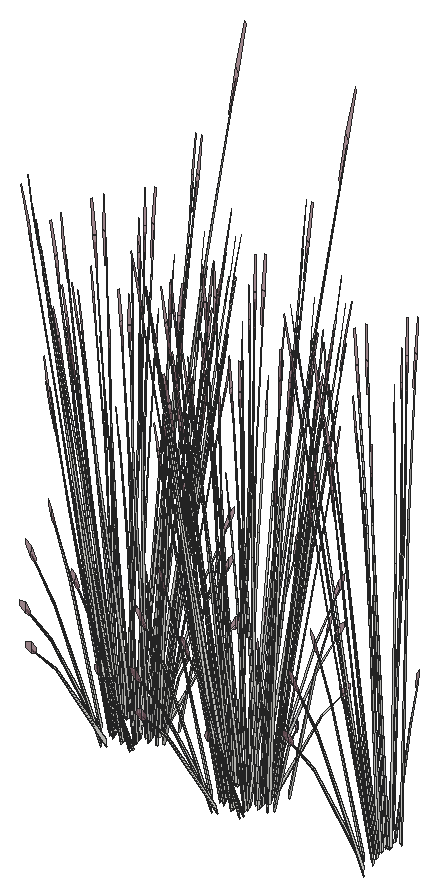
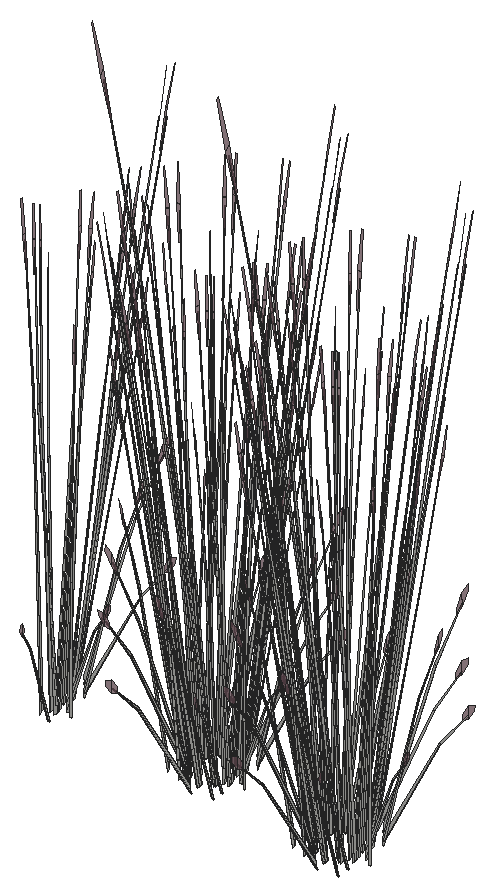
# SketchUp Ruby script. Lengths in inches.
U = 1.inch
M = Sketchup.active_model
def pt(a) = Geom::Point3d.new(a.map { |v| v * U })
def face(e, loops, mat)
  f = e.add_face(loops[0].map { |a| pt(a) })
  loops[1..].each { |l| e.add_face(l.map { |a| pt(a) }).erase! }
  f.material = f.back_material = mat if mat
  f
end
# faces: each face lists its corners as indices into pts; further lists are holes
def faces(e, pts, list, mat = nil) = list.each { |f| face(e, (f[0].is_a?(Array) ? f : [f]).map { |l| l.map { |i| pts[i] } }, mat) }
# xy, xz, yz: faces in a plane at the given z, y or x. An outline is a flat list of corners, or four numbers for a rectangle; further outlines are holes
def ring(l) = l.size == 4 ? [[l[0], l[1]], [l[2], l[1]], [l[2], l[3]], [l[0], l[3]]] : l.each_slice(2).to_a
def flat(e, list, mat, &to3) = list.each { |f| face(e, (f[0].is_a?(Array) ? f : [f]).map { |l| ring(l).map { |u, v| to3.(u, v) } }, mat) }
def xy(e, z, list, mat = nil) = flat(e, list, mat) { |x, y| [x, y, z] }
def xz(e, y, list, mat = nil) = flat(e, list, mat) { |x, z| [x, y, z] }
def yz(e, x, list, mat = nil) = flat(e, list, mat) { |y, z| [x, y, z] }
def lines(e, pts, list) = list.each { |a, b| e.add_line(pt(pts[a]), pt(pts[b])) }
# prism: a flat outline (further loops are holes) pulled along v
def prism(e, loops, v, mat = nil)
  f = face(e, loops, mat); d = Geom::Vector3d.new(v.map { |x| x * U })
  f.pushpull(f.normal.samedirection?(d) ? d.length : -d.length)
end
def box(e, o, s, mat = nil) = prism(e, [[o, [o[0] + s[0], o[1], o[2]], [o[0] + s[0], o[1] + s[1], o[2]], [o[0], o[1] + s[1], o[2]]]], [0, 0, s[2]], mat)
def at(x, y, z, deg = 0) = Geom::Transformation.translation(pt([x, y, z])) * Geom::Transformation.rotation(ORIGIN, Z_AXIS, deg.degrees)
def axes(o, x, y, z) = Geom::Transformation.new([*x, 0, *y, 0, *z, 0, *pt(o).to_a, 1])
def part(name) = M.definitions.add(name)
# library, detail: a bought-in or finely detailed component or shape, given as its bounding box
def library(name, o, s) = part(name).tap { |d| box(d.entities, o, s) }
def detail(e, o, s) = box(e.add_group.entities, o, s)
def put(e, d, t, mat = nil) = e.add_instance(d, t).tap { |i| i.material = mat if mat }
def group(e, t, mat = nil) = e.add_group.tap { |g| g.transformation = t; g.material = mat if mat }.entities
root = M.entities
M.materials.add("LightPink_Translucent").color = [144, 107, 117]
M.materials["LightPink_Translucent"].alpha = 0.75
c1 = part("blade")
p = [[2.15,0.21,22],[0,0.17,0],[0.09,0.45,0],[2.18,0.31,22],[2.29,0.31,22],[0.38,0.45,0],
  [2.48,0.24,33],[2.49,0.24,33],[2.48,0.22,33]]
faces(c1.entities,p,[[0,1,2,3],[4,5,2,3],[6,3,4,7],[8,0,3,6]])
c2 = part("seeds")
p = [[0.3,-0.1,1.38],[-0.01,-0.03,1.59],[-0.01,-0.03,0.03],[0.14,-0.07,-0.07],[0.29,-0.03,3],[0.15,0.01,3.11]]
faces(c2.entities,p,[[0,1,2,3],[1,0,4,5]],"LightPink_Translucent")
c3 = part("blade with seeds")
put(c3.entities,c1,at(0,0,0))
put(c3.entities,c2,axes([2.4,0.25,30.99],[1.5799,-0.05474,1.17369],[-0.12525,1.92788,0.29478],[-0.07173,-0.02425,1.56792]))
put(root,c3,axes([341.86,791.42,4.72],[-0.05763,0.06055,1.74944],[0.0049,0.44239,-0.27667],[-0.13211,0.05753,0.14031]))
put(root,c3,axes([341.22,791.87,4.71],[0.04504,0.01251,1.77383],[0.13934,0.41205,-0.16761],[-0.0922,0.10815,0.31391]))
put(root,c3,axes([342.13,789.58,4.71],[0.02617,0.04654,1.77383],[-0.12614,0.41836,-0.16761],[-0.12775,0.00303,0.31391]))
put(root,c3,axes([342.42,789.3,4.72],[-0.07594,-0.00329,1.74944],[-0.24177,0.32918,-0.27667],[-0.129,-0.06726,0.14031]))
put(root,c3,axes([342.11,791.12,4.73],[0.09971,-0.42522,0.48003],[0.32782,0.1454,0.3958],[-0.12892,0.02555,0.9933]))
put(root,c3,axes([342.23,791,5.03],[0.17758,0.42229,-0.1216],[-0.31518,0.20752,-0.67495],[-0.13282,0.05572,1.02557]))
put(root,c3,axes([342.63,790.12,5.03],[-0.0189,0.47427,-0.1216],[-0.35781,-0.01296,-0.67495],[-0.13781,-0.03295,1.02557]))
put(root,c3,axes([342.09,791.01,4.73],[-0.12963,-0.31798,0.0643],[0.23638,-0.15564,0.50621],[-0.1042,0.03071,0.77189]))
put(root,c3,axes([342.19,792.18,4.73],[-0.08753,-0.42921,0.48003],[0.34336,-0.07449,0.3958],[-0.1012,0.10094,0.9933]))
put(root,c3,axes([342.37,790.04,5.09],[0.29147,-0.34417,0.53763],[0.25138,0.3655,0.4433],[-0.13675,-0.06349,1.11249]))
put(root,c3,axes([342.12,792.1,4.73],[-0.2423,-0.19613,0.0643],[0.14107,-0.2793,0.50621],[-0.07768,0.0903,0.77189]))
put(root,c3,axes([342.35,791.125,5.05],[0.29332,0.1301,0.35414],[-0.08555,0.37955,-0.4572],[-0.11809,0.0348,0.87481]))
put(root,c3,axes([342.5,790.04,4.73],[0.01777,-0.35463,0.0643],[0.26836,0.00972,0.50621],[-0.1028,-0.03711,0.77189]))
put(root,c3,axes([341.87,793.07,4.72],[-0.00877,0.09229,1.74944],[0.24897,0.32105,-0.27667],[-0.06518,0.15182,0.14031]))
put(root,c3,axes([343.33,789.43,5.43],[-0.23555,0.44708,-0.13619],[-0.34112,-0.25757,-0.75594],[-0.11858,-0.12631,1.14864]))
put(root,c3,axes([342.68,790.31,5.05],[0.20082,0.29199,0.35414],[-0.2293,0.2764,-0.4572],[-0.1165,-0.04206,0.87481]))
put(root,c3,axes([342.24,792,5.03],[0.32648,0.25715,-0.1216],[-0.18809,0.3724,-0.67495],[-0.09224,0.12945,1.02557]))
put(root,c3,axes([341.7,793.12,5.65],[0.31145,0.12449,-0.06488],[-0.0958,0.38314,-0.29416],[-0.05094,0.05817,0.97024]))
put(root,c3,axes([342.4,792.04,5.05],[0.30722,-0.06665,0.35414],[0.08112,0.381,-0.4572],[-0.08804,0.10234,0.87481]))
put(root,c3,axes([343.23,788.36,4.71],[-0.00658,0.0559,1.77383],[-0.32474,0.20287,-0.16761],[-0.09556,-0.1037,0.31391]))
put(root,c3,axes([342.69,793.05,4.73],[-0.25132,-0.3182,0.48003],[0.2669,-0.27442,0.3958],[-0.04636,0.14929,0.9933]))
put(root,c3,axes([342.6,793.02,4.73],[-0.29004,-0.02173,0.0643],[0.00795,-0.32812,0.50621],[-0.03035,0.12569,0.77189]))
put(root,c3,axes([343.3,789.8,5.05],[0.05451,0.37564,0.35414],[-0.31161,0.09919,-0.4572],[-0.0837,-0.10765,0.87481]))
put(root,c3,axes([341.84,794.02,4.71],[0.04004,-0.02816,1.77383],[0.33095,0.18728,-0.16761],[-0.00778,0.15594,0.31391]))
put(root,c3,axes([343.16,789.36,5.09],[0.39316,-0.11987,0.53763],[0.06823,0.47021,0.4433],[-0.09247,-0.13858,1.11249]))
put(root,c3,axes([343.25,789.46,4.73],[0.16041,-0.29625,0.0643],[0.22843,0.17248,0.50621],[-0.07385,-0.09498,0.77189]))
put(root,c3,axes([343.6,788.58,4.72],[-0.05398,-0.06539,1.74944],[-0.36026,0.04145,-0.27667],[-0.0575,-0.15639,0.14031]))
put(root,c3,axes([342.82,792.79,5.05],[0.23881,-0.24554,0.35414],[0.22606,0.28036,-0.4572],[-0.0344,0.14245,0.87481]))
put(root,c3,axes([342.66,792.86,5.4],[0.3879,0.02311,-0.13498],[-0.0106,0.43749,-0.74919],[-0.02694,0.1685,1.13838]))
put(root,c3,axes([344.15,789.59,5.03],[-0.34538,0.21713,-0.1216],[-0.16972,-0.38536,-0.67495],[-0.04557,-0.16239,1.02557]))
put(root,c3,axes([344.05,789.74,5.05],[-0.1064,0.35863,0.35414],[-0.31043,-0.1046,-0.4572],[-0.02846,-0.14439,0.87481]))
put(root,c3,axes([343.48,793.49,5.0625],[-0.34777,-0.12192,0.53283],[0.11892,-0.40083,0.43934],[0.0209,0.15763,1.10256]))
put(root,c3,axes([343.39,793.52,4.73],[-0.26007,0.1585,0.0643],[-0.12729,-0.28902,0.50621],[0.02512,0.1274,0.77189]))
put(root,c3,axes([344.14,789.41,4.73],[0.26007,-0.1585,0.0643],[0.12729,0.28902,0.50621],[-0.02512,-0.1274,0.77189]))
put(root,c3,axes([343.3,794.21,4.72],[0.04474,0.0751,1.74944],[0.36104,0.0295,-0.27667],[0.03631,0.16562,0.14031]))
put(root,c3,axes([344.05,789.44,4.73],[0.34777,0.12192,0.48003],[-0.11892,0.40083,0.3958],[-0.0209,-0.15763,0.9933]))
put(root,c3,axes([343.49,793.2,5.05],[0.1064,-0.35863,0.35414],[0.31043,0.1046,-0.4572],[0.02846,0.14439,0.87481]))
put(root,c3,axes([343.9,794.48,5.65],[0.2439,-0.26754,-0.06488],[0.22348,0.29302,-0.29416],[0.01573,0.08303,0.97024]))
put(root,c3,axes([343.38,793.35,5.03],[0.34538,-0.21713,-0.1216],[0.16972,0.38536,-0.67495],[0.04557,0.16239,1.02557]))
put(root,c3,axes([345.15,789.05,4.71],[-0.03584,0.03562,1.77383],[-0.35118,-0.12018,-0.16761],[-0.01271,-0.15545,0.31391]))
put(root,c3,axes([344.87,790.08,5.03],[-0.3879,-0.02311,-0.1216],[0.0106,-0.43749,-0.67495],[0.02694,-0.1685,1.02557]))
put(root,c3,axes([344.72,790.14,5.05],[-0.23881,0.24554,0.35414],[-0.22606,-0.28036,-0.4572],[0.0344,-0.14245,0.87481]))
put(root,c3,axes([344.35,793.4,4.73],[-0.35104,0.10702,0.48003],[-0.06092,-0.41983,0.3958],[0.08256,0.12373,0.9933]))
put(root,c3,axes([344.28,793.48,4.73],[-0.16041,0.29625,0.0643],[-0.22843,-0.17248,0.50621],[0.07385,0.09498,0.77189]))
put(root,c3,axes([344.23,793.14,5.05],[-0.05451,-0.37564,0.35414],[0.31161,-0.09919,-0.4572],[0.0837,0.10765,0.87481]))
put(root,c3,axes([344.44,790.98,4.47],[-0.30498,-0.24231,1.38283],[0.32203,-0.37727,0.59665],[0.0984,0.22736,1.33663]))
put(root,c3,axes([343.93,793.66,4.71],[0.00104,-0.05646,1.77383],[0.30246,-0.2491,-0.16761],[0.10506,0.08891,0.31391]))
put(root,c3,axes([344.93,789.92,4.73],[0.29004,0.02173,0.0643],[-0.00795,0.32812,0.50621],[0.03035,-0.12569,0.77189]))
put(root,c3,axes([345.22,789.38,4.72],[-0.00341,-0.09282,1.74944],[-0.28775,-0.26825,-0.27667],[0.04449,-0.16261,0.14031]))
put(root,c3,axes([344.84,789.89,4.73],[0.25132,0.3182,0.48003],[-0.2669,0.27442,0.3958],[0.04636,-0.14929,0.9933]))
put(root,c3,axes([345.13,790.9,5.05],[-0.30722,0.06665,0.35414],[-0.08112,-0.381,-0.4572],[0.08804,-0.10234,0.87481]))
put(root,c3,axes([344.2,793.33,5.03],[0.21031,-0.39918,-0.1216],[0.30457,0.22997,-0.67495],[0.10587,0.11278,1.02557]))
put(root,c3,axes([345.29,790.9375,5.03],[-0.32648,-0.25715,-0.1216],[0.18809,-0.3724,-0.67495],[0.09224,-0.12945,1.02557]))
put(root,c3,axes([344.85,792.63,5.05],[-0.20082,-0.29199,0.35414],[0.2293,-0.2764,-0.4572],[0.1165,0.04206,0.87481]))
put(root,c3,axes([345.03,792.9,4.73],[-0.01777,0.35463,0.0643],[-0.26836,-0.00972,0.50621],[0.1028,0.03711,0.77189]))
put(root,c3,axes([345.06,792.78,4.73],[-0.26024,0.30729,0.48003],[-0.22444,-0.32634,0.3958],[0.1221,0.05668,0.9933]))
put(root,c3,axes([345.18,791.8125,5.05],[-0.29332,-0.1301,0.35414],[0.08555,-0.37955,-0.4572],[0.11809,-0.0348,0.87481]))
put(root,c3,axes([345.41,790.84,4.73],[0.2423,0.19613,0.0643],[-0.14107,0.2793,0.50621],[0.07768,-0.0903,0.77189]))
put(root,c3,axes([345.34,790.76,4.73],[0.08753,0.42921,0.48003],[-0.34336,0.07449,0.3958],[0.1012,-0.10094,0.9933]))
put(root,c3,axes([346.1,790.82,4.71],[-0.0461,-0.00354,1.77383],[-0.19143,-0.37951,-0.16761],[0.07688,-0.12478,0.31391]))
put(root,c3,axes([345.45,791.93,4.73],[0.12963,0.31798,0.0643],[-0.23638,0.15564,0.50621],[0.1042,-0.03071,0.77189]))
put(root,c3,axes([344.91,792.82,5.03],[0.0189,-0.47427,-0.1216],[0.35781,0.01296,-0.67495],[0.13781,0.03295,1.02557]))
put(root,c3,axes([345.31,791.94,5.03],[-0.17758,-0.42229,-0.1216],[0.31518,-0.20752,-0.67495],[0.13282,-0.05572,1.02557]))
put(root,c3,axes([345.42,791.82,4.73],[-0.09971,0.42522,0.48003],[-0.32782,-0.1454,0.3958],[0.12892,-0.02555,0.9933]))
put(root,c3,axes([345.22,792.53,4.72],[0.07571,-0.00789,1.74944],[0.20767,-0.36231,-0.27667],[0.13467,0.04783,0.14031]))
put(root,c3,axes([346.01,793.19,4.71],[-0.03191,-0.04083,1.77383],[0.06981,-0.43764,-0.16761],[0.12571,-0.02796,0.31391]))
put(root,c3,axes([346.27,791.28,4.72],[0.04898,-0.07104,1.74944],[-0.06269,-0.43574,-0.27667],[0.12289,-0.08262,0.14031]))
put(root,c3,axes([353.11,788.95,4.72],[-0.05763,0.06055,1.74944],[0.0049,0.44239,-0.27667],[-0.13211,0.05753,0.14031]))
put(root,c3,axes([352.47,789.39,4.71],[0.04504,0.01251,1.77383],[0.13934,0.41205,-0.16761],[-0.0922,0.10815,0.31391]))
put(root,c3,axes([353.38,787.1,4.71],[0.02617,0.04654,1.77383],[-0.12614,0.41836,-0.16761],[-0.12775,0.00303,0.31391]))
put(root,c3,axes([353.67,786.83,4.72],[-0.07594,-0.00329,1.74944],[-0.24177,0.32918,-0.27667],[-0.129,-0.06726,0.14031]))
put(root,c3,axes([353.36,788.65,4.73],[0.09971,-0.42522,0.48003],[0.32782,0.1454,0.3958],[-0.12892,0.02555,0.9933]))
put(root,c3,axes([353.48,788.52,5.03],[0.17758,0.42229,-0.1216],[-0.31518,0.20752,-0.67495],[-0.13282,0.05572,1.02557]))
put(root,c3,axes([353.88,787.65,5.03],[-0.0189,0.47427,-0.1216],[-0.35781,-0.01296,-0.67495],[-0.13781,-0.03295,1.02557]))
put(root,c3,axes([353.34,788.53,4.73],[-0.12963,-0.31798,0.0643],[0.23638,-0.15564,0.50621],[-0.1042,0.03071,0.77189]))
put(root,c3,axes([353.44,789.71,4.73],[-0.08753,-0.42921,0.48003],[0.34336,-0.07449,0.3958],[-0.1012,0.10094,0.9933]))
put(root,c3,axes([353.62,787.57,5.09],[0.29147,-0.34417,0.53763],[0.25138,0.3655,0.4433],[-0.13675,-0.06349,1.11249]))
put(root,c3,axes([353.375,789.625,4.73],[-0.2423,-0.19613,0.0643],[0.14107,-0.2793,0.50621],[-0.07768,0.0903,0.77189]))
put(root,c3,axes([353.6,788.65,5.05],[0.29332,0.1301,0.35414],[-0.08555,0.37955,-0.4572],[-0.11809,0.0348,0.87481]))
put(root,c3,axes([353.75,787.57,4.73],[0.01777,-0.35463,0.0643],[0.26836,0.00972,0.50621],[-0.1028,-0.03711,0.77189]))
put(root,c3,axes([353.12,790.6,4.72],[-0.00877,0.09229,1.74944],[0.24897,0.32105,-0.27667],[-0.06518,0.15182,0.14031]))
put(root,c3,axes([354.58,786.95,5.43],[-0.23555,0.44708,-0.13619],[-0.34112,-0.25757,-0.75594],[-0.11858,-0.12631,1.14864]))
put(root,c3,axes([353.93,787.83,5.05],[0.20082,0.29199,0.35414],[-0.2293,0.2764,-0.4572],[-0.1165,-0.04206,0.87481]))
put(root,c3,axes([353.49,789.53,5.03],[0.32648,0.25715,-0.1216],[-0.18809,0.3724,-0.67495],[-0.09224,0.12945,1.02557]))
put(root,c3,axes([352.95,790.64,5.65],[0.31145,0.12449,-0.06488],[-0.0958,0.38314,-0.29416],[-0.05094,0.05817,0.97024]))
put(root,c3,axes([353.65,789.5625,5.05],[0.30722,-0.06665,0.35414],[0.08112,0.381,-0.4572],[-0.08804,0.10234,0.87481]))
put(root,c3,axes([354.49,785.89,4.71],[-0.00658,0.0559,1.77383],[-0.32474,0.20287,-0.16761],[-0.09556,-0.1037,0.31391]))
put(root,c3,axes([353.94,790.57,4.73],[-0.25132,-0.3182,0.48003],[0.2669,-0.27442,0.3958],[-0.04636,0.14929,0.9933]))
put(root,c3,axes([353.85,790.54,4.73],[-0.29004,-0.02173,0.0643],[0.00795,-0.32812,0.50621],[-0.03035,0.12569,0.77189]))
put(root,c3,axes([354.55,787.33,5.05],[0.05451,0.37564,0.35414],[-0.31161,0.09919,-0.4572],[-0.0837,-0.10765,0.87481]))
put(root,c3,axes([353.09,791.54,4.71],[0.04004,-0.02816,1.77383],[0.33095,0.18728,-0.16761],[-0.00778,0.15594,0.31391]))
put(root,c3,axes([354.41,786.88,5.09],[0.39316,-0.11987,0.53763],[0.06823,0.47021,0.4433],[-0.09247,-0.13858,1.11249]))
put(root,c3,axes([354.51,786.99,4.73],[0.16041,-0.29625,0.0643],[0.22843,0.17248,0.50621],[-0.07385,-0.09498,0.77189]))
put(root,c3,axes([354.86,786.11,4.72],[-0.05398,-0.06539,1.74944],[-0.36026,0.04145,-0.27667],[-0.0575,-0.15639,0.14031]))
put(root,c3,axes([354.07,790.32,5.05],[0.23881,-0.24554,0.35414],[0.22606,0.28036,-0.4572],[-0.0344,0.14245,0.87481]))
put(root,c3,axes([353.91,790.39,5.4],[0.3879,0.02311,-0.13498],[-0.0106,0.43749,-0.74919],[-0.02694,0.1685,1.13838]))
put(root,c3,axes([355.4,787.11,5.03],[-0.34538,0.21713,-0.1216],[-0.16972,-0.38536,-0.67495],[-0.04557,-0.16239,1.02557]))
put(root,c3,axes([355.3,787.27,5.05],[-0.1064,0.35863,0.35414],[-0.31043,-0.1046,-0.4572],[-0.02846,-0.14439,0.87481]))
put(root,c3,axes([354.73,791.02,5.0625],[-0.34777,-0.12192,0.53283],[0.11892,-0.40083,0.43934],[0.0209,0.15763,1.10256]))
put(root,c3,axes([354.64,791.05,4.73],[-0.26007,0.1585,0.0643],[-0.12729,-0.28902,0.50621],[0.02512,0.1274,0.77189]))
put(root,c3,axes([355.4,786.94,4.73],[0.26007,-0.1585,0.0643],[0.12729,0.28902,0.50621],[-0.02512,-0.1274,0.77189]))
put(root,c3,axes([354.55,791.74,4.72],[0.04474,0.0751,1.74944],[0.36104,0.0295,-0.27667],[0.03631,0.16562,0.14031]))
put(root,c3,axes([355.3,786.97,4.73],[0.34777,0.12192,0.48003],[-0.11892,0.40083,0.3958],[-0.0209,-0.15763,0.9933]))
put(root,c3,axes([354.74,790.73,5.05],[0.1064,-0.35863,0.35414],[0.31043,0.1046,-0.4572],[0.02846,0.14439,0.87481]))
put(root,c3,axes([355.15,792.01,5.65],[0.2439,-0.26754,-0.06488],[0.22348,0.29302,-0.29416],[0.01573,0.08303,0.97024]))
put(root,c3,axes([354.63,790.875,5.03],[0.34538,-0.21713,-0.1216],[0.16972,0.38536,-0.67495],[0.04557,0.16239,1.02557]))
put(root,c3,axes([356.4,786.57,4.71],[-0.03584,0.03562,1.77383],[-0.35118,-0.12018,-0.16761],[-0.01271,-0.15545,0.31391]))
put(root,c3,axes([356.12,787.6,5.03],[-0.3879,-0.02311,-0.1216],[0.0106,-0.43749,-0.67495],[0.02694,-0.1685,1.02557]))
put(root,c3,axes([355.97,787.67,5.05],[-0.23881,0.24554,0.35414],[-0.22606,-0.28036,-0.4572],[0.0344,-0.14245,0.87481]))
put(root,c3,axes([355.6,790.92,4.73],[-0.35104,0.10702,0.48003],[-0.06092,-0.41983,0.3958],[0.08256,0.12373,0.9933]))
put(root,c3,axes([355.53,791.01,4.73],[-0.16041,0.29625,0.0643],[-0.22843,-0.17248,0.50621],[0.07385,0.09498,0.77189]))
put(root,c3,axes([355.48,790.67,5.05],[-0.05451,-0.37564,0.35414],[0.31161,-0.09919,-0.4572],[0.0837,0.10765,0.87481]))
put(root,c3,axes([355.69,788.51,4.47],[-0.30498,-0.24231,1.38283],[0.32203,-0.37727,0.59665],[0.0984,0.22736,1.33663]))
put(root,c3,axes([355.18,791.19,4.71],[0.00104,-0.05646,1.77383],[0.30246,-0.2491,-0.16761],[0.10506,0.08891,0.31391]))
put(root,c3,axes([356.1875,787.45,4.73],[0.29004,0.02173,0.0643],[-0.00795,0.32812,0.50621],[0.03035,-0.12569,0.77189]))
put(root,c3,axes([356.47,786.91,4.72],[-0.00341,-0.09282,1.74944],[-0.28775,-0.26825,-0.27667],[0.04449,-0.16261,0.14031]))
put(root,c3,axes([356.09,787.42,4.73],[0.25132,0.3182,0.48003],[-0.2669,0.27442,0.3958],[0.04636,-0.14929,0.9933]))
put(root,c3,axes([356.38,788.43,5.05],[-0.30722,0.06665,0.35414],[-0.08112,-0.381,-0.4572],[0.08804,-0.10234,0.87481]))
put(root,c3,axes([355.45,790.86,5.03],[0.21031,-0.39918,-0.1216],[0.30457,0.22997,-0.67495],[0.10587,0.11278,1.02557]))
put(root,c3,axes([356.54,788.46,5.03],[-0.32648,-0.25715,-0.1216],[0.18809,-0.3724,-0.67495],[0.09224,-0.12945,1.02557]))
put(root,c3,axes([356.1,790.16,5.05],[-0.20082,-0.29199,0.35414],[0.2293,-0.2764,-0.4572],[0.1165,0.04206,0.87481]))
put(root,c3,axes([356.28,790.42,4.73],[-0.01777,0.35463,0.0643],[-0.26836,-0.00972,0.50621],[0.1028,0.03711,0.77189]))
put(root,c3,axes([356.31,790.3125,4.73],[-0.26024,0.30729,0.48003],[-0.22444,-0.32634,0.3958],[0.1221,0.05668,0.9933]))
put(root,c3,axes([356.43,789.34,5.05],[-0.29332,-0.1301,0.35414],[0.08555,-0.37955,-0.4572],[0.11809,-0.0348,0.87481]))
put(root,c3,axes([356.66,788.37,4.73],[0.2423,0.19613,0.0643],[-0.14107,0.2793,0.50621],[0.07768,-0.0903,0.77189]))
put(root,c3,axes([356.59,788.29,4.73],[0.08753,0.42921,0.48003],[-0.34336,0.07449,0.3958],[0.1012,-0.10094,0.9933]))
put(root,c3,axes([357.35,788.35,4.71],[-0.0461,-0.00354,1.77383],[-0.19143,-0.37951,-0.16761],[0.07688,-0.12478,0.31391]))
put(root,c3,axes([356.7,789.46,4.73],[0.12963,0.31798,0.0643],[-0.23638,0.15564,0.50621],[0.1042,-0.03071,0.77189]))
put(root,c3,axes([356.16,790.34,5.03],[0.0189,-0.47427,-0.1216],[0.35781,0.01296,-0.67495],[0.13781,0.03295,1.02557]))
put(root,c3,axes([356.56,789.47,5.03],[-0.17758,-0.42229,-0.1216],[0.31518,-0.20752,-0.67495],[0.13282,-0.05572,1.02557]))
put(root,c3,axes([356.67,789.35,4.73],[-0.09971,0.42522,0.48003],[-0.32782,-0.1454,0.3958],[0.12892,-0.02555,0.9933]))
put(root,c3,axes([356.47,790.06,4.72],[0.07571,-0.00789,1.74944],[0.20767,-0.36231,-0.27667],[0.13467,0.04783,0.14031]))
put(root,c3,axes([357.26,790.72,4.71],[-0.03191,-0.04083,1.77383],[0.06981,-0.43764,-0.16761],[0.12571,-0.02796,0.31391]))
put(root,c3,axes([357.52,788.81,4.72],[0.04898,-0.07104,1.74944],[-0.06269,-0.43574,-0.27667],[0.12289,-0.08262,0.14031]))
put(root,c3,axes([366.1875,788.59,4.72],[-0.05763,0.06055,1.74944],[0.0049,0.44239,-0.27667],[-0.13211,0.05753,0.14031]))
put(root,c3,axes([365.55,789.04,4.71],[0.04504,0.01251,1.77383],[0.13934,0.41205,-0.16761],[-0.0922,0.10815,0.31391]))
put(root,c3,axes([366.46,786.75,4.71],[0.02617,0.04654,1.77383],[-0.12614,0.41836,-0.16761],[-0.12775,0.00303,0.31391]))
put(root,c3,axes([366.75,786.47,4.72],[-0.07594,-0.00329,1.74944],[-0.24177,0.32918,-0.27667],[-0.129,-0.06726,0.14031]))
put(root,c3,axes([366.44,788.29,4.73],[0.09971,-0.42522,0.48003],[0.32782,0.1454,0.3958],[-0.12892,0.02555,0.9933]))
put(root,c3,axes([366.56,788.17,5.03],[0.17758,0.42229,-0.1216],[-0.31518,0.20752,-0.67495],[-0.13282,0.05572,1.02557]))
put(root,c3,axes([366.96,787.29,5.03],[-0.0189,0.47427,-0.1216],[-0.35781,-0.01296,-0.67495],[-0.13781,-0.03295,1.02557]))
put(root,c3,axes([366.42,788.18,4.73],[-0.12963,-0.31798,0.0643],[0.23638,-0.15564,0.50621],[-0.1042,0.03071,0.77189]))
put(root,c3,axes([366.52,789.35,4.73],[-0.08753,-0.42921,0.48003],[0.34336,-0.07449,0.3958],[-0.1012,0.10094,0.9933]))
put(root,c3,axes([366.7,787.22,5.09],[0.29147,-0.34417,0.53763],[0.25138,0.3655,0.4433],[-0.13675,-0.06349,1.11249]))
put(root,c3,axes([366.45,789.27,4.73],[-0.2423,-0.19613,0.0643],[0.14107,-0.2793,0.50621],[-0.07768,0.0903,0.77189]))
put(root,c3,axes([366.68,788.3,5.05],[0.29332,0.1301,0.35414],[-0.08555,0.37955,-0.4572],[-0.11809,0.0348,0.87481]))
put(root,c3,axes([366.83,787.21,4.73],[0.01777,-0.35463,0.0643],[0.26836,0.00972,0.50621],[-0.1028,-0.03711,0.77189]))
put(root,c3,axes([366.2,790.24,4.72],[-0.00877,0.09229,1.74944],[0.24897,0.32105,-0.27667],[-0.06518,0.15182,0.14031]))
put(root,c3,axes([367.66,786.6,5.43],[-0.23555,0.44708,-0.13619],[-0.34112,-0.25757,-0.75594],[-0.11858,-0.12631,1.14864]))
put(root,c3,axes([367.01,787.48,5.05],[0.20082,0.29199,0.35414],[-0.2293,0.2764,-0.4572],[-0.1165,-0.04206,0.87481]))
put(root,c3,axes([366.57,789.17,5.03],[0.32648,0.25715,-0.1216],[-0.18809,0.3724,-0.67495],[-0.09224,0.12945,1.02557]))
put(root,c3,axes([366.03,790.29,5.65],[0.31145,0.12449,-0.06488],[-0.0958,0.38314,-0.29416],[-0.05094,0.05817,0.97024]))
put(root,c3,axes([366.73,789.21,5.05],[0.30722,-0.06665,0.35414],[0.08112,0.381,-0.4572],[-0.08804,0.10234,0.87481]))
put(root,c3,axes([367.57,785.54,4.71],[-0.00658,0.0559,1.77383],[-0.32474,0.20287,-0.16761],[-0.09556,-0.1037,0.31391]))
put(root,c3,axes([367.02,790.22,4.73],[-0.25132,-0.3182,0.48003],[0.2669,-0.27442,0.3958],[-0.04636,0.14929,0.9933]))
